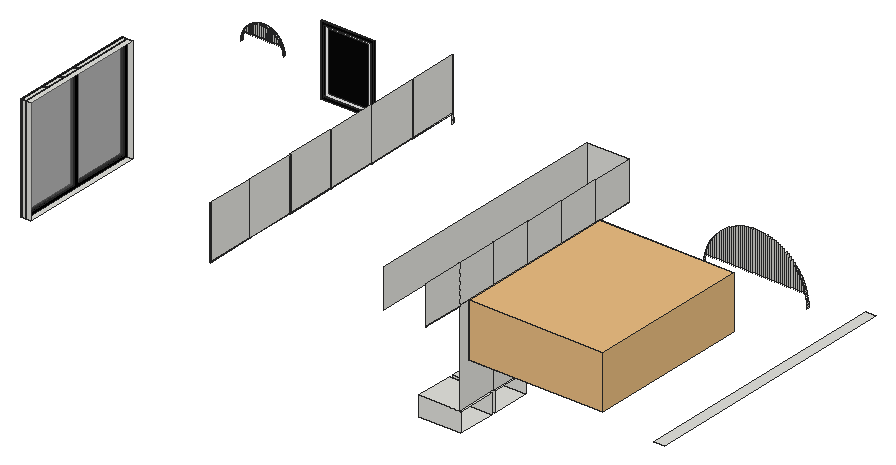
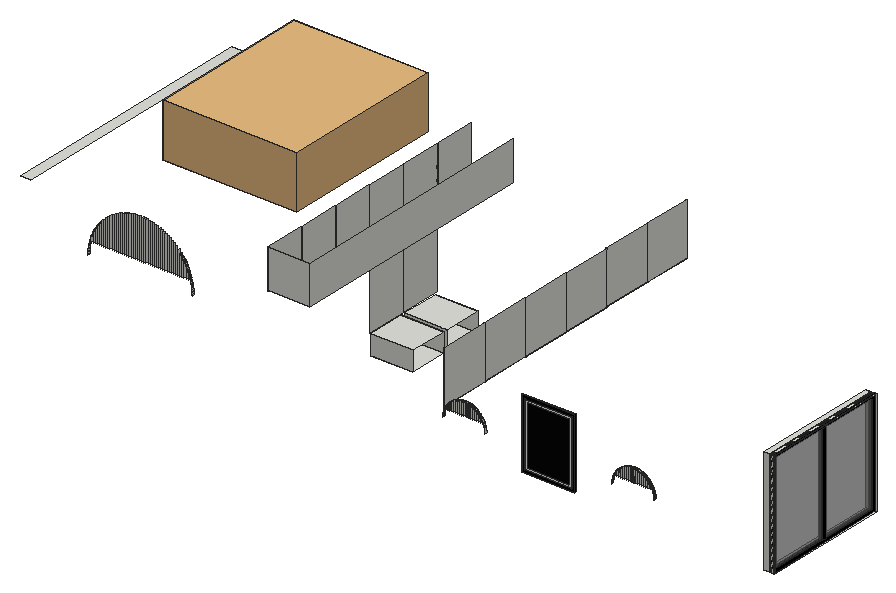
# SketchUp Ruby script. Lengths in inches.
U = 1.inch
M = Sketchup.active_model
def pt(a) = Geom::Point3d.new(a.map { |v| v * U })
def face(e, loops, mat)
  f = e.add_face(loops[0].map { |a| pt(a) })
  loops[1..].each { |l| e.add_face(l.map { |a| pt(a) }).erase! }
  f.material = f.back_material = mat if mat
  f
end
# faces: each face lists its corners as indices into pts; further lists are holes
def faces(e, pts, list, mat = nil) = list.each { |f| face(e, (f[0].is_a?(Array) ? f : [f]).map { |l| l.map { |i| pts[i] } }, mat) }
# xy, xz, yz: faces in a plane at the given z, y or x. An outline is a flat list of corners, or four numbers for a rectangle; further outlines are holes
def ring(l) = l.size == 4 ? [[l[0], l[1]], [l[2], l[1]], [l[2], l[3]], [l[0], l[3]]] : l.each_slice(2).to_a
def flat(e, list, mat, &to3) = list.each { |f| face(e, (f[0].is_a?(Array) ? f : [f]).map { |l| ring(l).map { |u, v| to3.(u, v) } }, mat) }
def xy(e, z, list, mat = nil) = flat(e, list, mat) { |x, y| [x, y, z] }
def xz(e, y, list, mat = nil) = flat(e, list, mat) { |x, z| [x, y, z] }
def yz(e, x, list, mat = nil) = flat(e, list, mat) { |y, z| [x, y, z] }
def lines(e, pts, list) = list.each { |a, b| e.add_line(pt(pts[a]), pt(pts[b])) }
# prism: a flat outline (further loops are holes) pulled along v
def prism(e, loops, v, mat = nil)
  f = face(e, loops, mat); d = Geom::Vector3d.new(v.map { |x| x * U })
  f.pushpull(f.normal.samedirection?(d) ? d.length : -d.length)
end
def box(e, o, s, mat = nil) = prism(e, [[o, [o[0] + s[0], o[1], o[2]], [o[0] + s[0], o[1] + s[1], o[2]], [o[0], o[1] + s[1], o[2]]]], [0, 0, s[2]], mat)
def at(x, y, z, deg = 0) = Geom::Transformation.translation(pt([x, y, z])) * Geom::Transformation.rotation(ORIGIN, Z_AXIS, deg.degrees)
def axes(o, x, y, z) = Geom::Transformation.new([*x, 0, *y, 0, *z, 0, *pt(o).to_a, 1])
def part(name) = M.definitions.add(name)
# library, detail: a bought-in or finely detailed component or shape, given as its bounding box
def library(name, o, s) = part(name).tap { |d| box(d.entities, o, s) }
def detail(e, o, s) = box(e.add_group.entities, o, s)
def put(e, d, t, mat = nil) = e.add_instance(d, t).tap { |i| i.material = mat if mat }
def group(e, t, mat = nil) = e.add_group.tap { |g| g.transformation = t; g.material = mat if mat }.entities
root = M.entities
M.materials.add("Plastic_Metalic_Black").color = [8, 8, 8]
M.materials.add("[Color M00]1").color = [254, 254, 254]
M.materials.add("[Color_008]").color = [30, 30, 30]
M.materials.add("[Color_009]").color = [0, 0, 0]
M.materials.add("[Translucent_Glass_Gray]").color = [128, 128, 128]
M.materials["[Translucent_Glass_Gray]"].alpha = 0.5
c1 = part("Photos Gallery Wall")
g1 = group(c1.entities,at(0,0,0))
xy(g1,23.66,[[13.71,0.34,13.7,1.03,31.9375,1.12,31.94,0.43]],"Plastic_Metalic_Black")
xy(g1,24.66,[[14.71,0.34,30.94,0.42,30.9375,1.02,14.7,0.94]],"Plastic_Metalic_Black")
xy(g1,48.82,[[14.71,0.34,14.7,0.94,30.9375,1.02,30.94,0.42]],"Plastic_Metalic_Black")
xy(g1,49.82,[[13.71,0.34,31.94,0.43,31.9375,1.12,13.7,1.03]],"Plastic_Metalic_Black")
p = [[13.7,1.03,49.82],[13.7,1.03,23.66],[13.71,0.34,23.66],[13.71,0.34,49.82],[31.94,0.43,23.66],[31.94,0.43,49.82],
  [30.94,0.42,24.66],[14.71,0.34,24.66],[14.71,0.34,48.82],[30.94,0.42,48.82],[31.9375,1.12,23.66],[31.9375,1.12,49.82],
  [14.7,1.04,24.66],[30.9375,1.11,24.66],[30.9375,1.11,48.82],[14.7,1.04,48.82],[14.7,0.94,48.82],[14.7,0.94,24.66],
  [30.9375,1.02,24.66],[30.9375,1.02,48.82],[29.9375,1.02,47.82],[29.9375,1.02,25.66],[15.7,0.95,25.66],[15.7,0.95,47.82]]
faces(g1,p,[[0,1,2,3],[[4,5,3,2],[6,7,8,9]],[10,11,5,4],[[11,10,1,0],[12,13,14,15]],[16,8,7,17],[18,6,9,19],[21,20,23,22]],"Plastic_Metalic_Black")
faces(g1,p,[[[17,18,19,16],[20,21,22,23]]],"[Color M00]1")
lines(g1,p,[[14,19],[15,16],[12,17],[13,18]])
c2 = part("Photo+Frames+03")
put(c2.entities,c1,axes([128.61,79.32,-32.19],[1.3608,0,0],[0,1.3608,0],[0,0,1.3608]))
c3 = library("ceiling fan",[0,0,0],[76.25,93.13,30.02])
xy(root,30.7,[[245.003,91.2,268.823,112.8],[245.003,115.2,268.823,136.8]])
xy(root,36,[[0,114.57,6,186.57]])
xy(root,41.7,[[245.003,91.2,268.823,112.8],[245.003,115.2,268.823,136.8]])
xy(root,88.8,[[150,61.77,150.18,89.203],[150,89.603,150.18,118.037],[150,118.437,150.18,146.87],[150,147.27,150.18,175.703],[150,176.103,150.18,204.537],
  [150,204.937,150.18,233.37]])
xy(root,89.2,[[150,61.77,150.18,89.203],[150,89.603,150.18,118.037],[150,118.437,150.18,146.87],[150,147.27,150.18,175.703],[150,176.103,150.18,204.537],
  [150,204.937,150.18,233.37]])
xy(root,95.8,[[268.823,66.2,269.003,89.8],[268.823,138.2,269.003,161.8],[268.823,162.2,269.003,185.8],[268.823,186.2,269.003,209.8]])
xy(root,96,[[413.003,48,419.003,198],[0,114.57,6,186.57]])
xy(root,96.2,[[268.823,66.2,269.003,89.8],[268.823,90.2,269.003,113.8],[268.823,114.2,269.003,137.8],[268.823,138.2,269.003,161.8],[268.823,162.2,269.003,185.8],
  [268.823,186.2,269.003,209.8]])
xz(root,61.77,[[150,89.2,150.18,118.8]])
xz(root,66.2,[[268.823,96.2,269.003,117.8]])
xz(root,89.203,[[150,89.2,150.18,118.8]])
xz(root,89.603,[[150,89.2,150.18,118.8]])
xz(root,89.8,[[268.823,96.2,269.003,117.8]])
xz(root,90.2,[[268.823,96.2,269.003,117.8]])
xz(root,91.2,[[245.003,30.7,268.823,41.7]])
xz(root,112.8,[[245.003,30.7,268.823,41.7]])
xz(root,113.8,[[268.823,96.2,269.003,117.8]])
xz(root,114.2,[[268.823,96.2,269.003,117.8]])
xz(root,114.57,[[0,36,6,96]])
xz(root,115.2,[[245.003,30.7,268.823,41.7]])
xz(root,118.037,[[150,89.2,150.18,118.8]])
xz(root,118.437,[[150,89.2,150.18,118.8]])
xz(root,136.8,[[245.003,30.7,268.823,41.7]])
xz(root,137.8,[[268.823,96.2,269.003,117.8]])
xz(root,138.2,[[268.823,96.2,269.003,117.8]])
xz(root,146.87,[[150,89.2,150.18,118.8]])
xz(root,147.27,[[150,89.2,150.18,118.8]])
xz(root,161.8,[[268.823,96.2,269.003,117.8]])
xz(root,162.2,[[268.823,96.2,269.003,117.8]])
xz(root,175.703,[[150,89.2,150.18,118.8]])
xz(root,176.103,[[150,89.2,150.18,118.8]])
xz(root,185.8,[[268.823,96.2,269.003,117.8]])
xz(root,186.2,[[268.823,96.2,269.003,117.8]])
xz(root,186.57,[[0,36,6,96]])
xz(root,204.537,[[150,89.2,150.18,118.8]])
xz(root,204.937,[[150,89.2,150.18,118.8]])
xz(root,209.8,[[268.823,96.2,269.003,117.8]])
xz(root,210,[[245.003,96,268.823,118]])
xz(root,233.37,[[150,84,150.18,88.8],[150,89.2,150.18,118.8]])
xz(root,233.57,[[150,84,150.18,119]])
xz(root,234.57,[[126,84,126.409,87.106,126.332,86.801,126.262,86.495,126.201,86.187,126.148,85.877,126.103,85.566,126.066,85.254,126.037,84.942,126.016,84.628,126.004,84.314],[126.409,87.106,127,88.533,127,88.794,126.913,88.592,126.797,88.3,126.688,88.006,126.587,87.708,126.494,87.408],[127,88.533,127.2,89.016,127.2,89.229,127.169,89.166,127.037,88.881,127,88.794],[127.2,89.016,127.608,90,128.2,90.772,128.2,90.924,128.11,90.797,127.936,90.536,127.768,90.27,127.608,90,127.454,89.726,127.308,89.448,127.2,89.229],[128.2,90.772,128.4,91.033,128.4,91.198,128.292,91.053,128.2,90.924],
  [128.4,91.033,129.4,92.336,129.4,92.368,129.296,92.26,129.082,92.03,128.875,91.793,128.674,91.552,128.48,91.305,128.4,91.198],[129.6,92.551,130.6,93.318,130.6,93.445,130.448,93.326,130.207,93.125,129.97,92.918,129.74,92.704,129.6,92.568],[130.6,93.318,130.8,93.472,130.8,93.599,130.695,93.52,130.6,93.445]])
yz(root,32.2,[[233.57,88.794,234.57,90.924]])
yz(root,32.4,[[233.57,89.229,234.57,91.198]])
yz(root,33.4,[[233.57,88.794,234.57,90.924],[233.57,90.924,234.57,92.368]])
yz(root,33.6,[[233.57,89.229,234.57,92.568]])
yz(root,34.6,[[233.57,88.794,234.57,89.229],[233.57,89.229,234.57,93.423],[233.57,93.423,234.57,93.445]])
yz(root,34.8,[[233.57,89.229,234.57,93.52],[233.57,93.52,234.57,93.599]])
yz(root,35.8,[[233.57,88.794,234.57,94.273]])
yz(root,36,[[233.57,89.229,234.57,94.392]])
yz(root,37,[[233.57,88.794,234.57,94.908]])
yz(root,37.2,[[233.57,89.229,234.57,94.997]])
yz(root,38.2,[[233.57,88.794,234.57,95.382]])
yz(root,38.4,[[233.57,89.229,234.57,95.446]])
yz(root,39.4,[[233.57,88.794,234.57,95.714]])
yz(root,39.6,[[233.57,89.229,234.57,95.757]])
yz(root,40.6,[[233.57,88.794,234.57,95.917]])
yz(root,41.8,[[233.57,88.794,234.57,95.997]])
yz(root,42,[[233.57,89.229,234.57,89.417],[233.57,89.417,234.57,96]])
yz(root,43,[[233.57,88.794,234.57,88.981],[233.57,88.981,234.57,95.958]])
yz(root,43.2,[[233.57,89.229,234.57,89.417],[233.57,89.417,234.57,95.939]])
yz(root,45.6,[[233.57,89.229,234.57,95.446]])
yz(root,48,[[233.57,89.229,234.57,94.392]])
yz(root,50.2,[[233.57,88.794,234.57,92.76]])
yz(root,50.4,[[233.695,89.229,234.57,92.568]])
yz(root,51.4,[[233.695,88.794,234.57,91.458]])
yz(root,51.6,[[233.695,89.229,234.57,91.198]])
yz(root,52.6,[[233.695,88.794,234.57,89.623]])
yz(root,128.2,[[233.57,88.794,234.57,90.772]])
yz(root,128.4,[[233.57,89.229,234.57,91.033]])
yz(root,129.4,[[233.57,88.794,234.57,90.924],[233.57,90.924,234.57,92.336]])
yz(root,129.6,[[233.57,89.229,234.57,92.551]])
yz(root,130.6,[[233.57,88.794,234.57,89.229],[233.57,89.229,234.57,93.318]])
yz(root,130.8,[[233.57,89.229,234.57,93.472],[233.57,93.472,234.57,93.52],[233.57,93.52,234.57,93.599]])
yz(root,131.8,[[233.57,88.794,234.57,94.273]])
yz(root,132,[[233.57,89.229,234.57,94.392]])
yz(root,133,[[233.57,88.794,234.57,94.908]])
yz(root,133.2,[[233.57,89.229,234.57,94.997]])
yz(root,134.2,[[233.57,88.794,234.57,95.382]])
yz(root,134.4,[[233.57,89.229,234.57,95.446]])
yz(root,135.4,[[233.57,88.794,234.57,95.714]])
yz(root,135.6,[[233.57,89.229,234.57,95.757]])
yz(root,136.6,[[233.57,88.794,234.57,95.917]])
yz(root,137.8,[[233.57,88.794,234.57,95.997]])
yz(root,138,[[233.57,89.229,234.57,89.417],[233.57,89.417,234.57,96]])
yz(root,139,[[233.57,88.794,234.57,88.981],[233.57,88.981,234.57,95.958]])
yz(root,139.2,[[233.57,89.229,234.57,89.417],[233.57,89.417,234.57,95.939]])
yz(root,141.6,[[233.57,89.229,234.57,95.446]])
yz(root,144,[[233.57,89.229,234.57,94.392]])
yz(root,146.2,[[233.57,88.794,234.57,92.76]])
yz(root,146.4,[[233.57,89.229,234.57,92.568]])
yz(root,147.4,[[233.57,88.794,234.57,91.458]])
yz(root,147.6,[[233.57,89.229,234.57,91.198]])
yz(root,148.6,[[233.57,88.794,234.57,89.623]])
yz(root,150,[[61.77,89.2,89.203,118.8],[89.603,89.2,118.037,118.8],[118.437,89.2,146.87,118.8],[147.27,89.2,175.703,118.8],[176.103,89.2,204.537,118.8],
  [204.937,89.2,233.37,118.8]])
yz(root,245.003,[[66,96,210,118]])
yz(root,268.823,[[90.2,42.7,113.8,95.8],[114.2,42.7,137.8,95.8]])
yz(root,269.003,[[66.2,96.2,89.8,117.8],[90.2,96.2,113.8,117.8],[114.2,96.2,137.8,117.8],[138.2,96.2,161.8,117.8],[162.2,96.2,185.8,117.8],
  [186.2,96.2,209.8,117.8]])
yz(root,313.953,[[209,85.483,210,89.103]])
yz(root,315.153,[[209,85.483,210,91.7]])
yz(root,316.353,[[208.6875,85.483,210,93.787]])
yz(root,317.553,[[209,85.483,210,95.548]])
yz(root,318.753,[[209,85.483,210,97.071]])
yz(root,319.953,[[209,85.483,210,98.413]])
yz(root,321.153,[[209,85.483,210,99.602]])
yz(root,322.353,[[209,85.483,210,100.667]])
yz(root,323.553,[[209,85.483,210,101.623]])
yz(root,324.753,[[209,85.483,210,102.484]])
yz(root,325.953,[[209,85.483,210,103.259]])
yz(root,327.153,[[209,85.483,210,103.954]])
yz(root,328.353,[[209,85.483,210,104.576]])
yz(root,329.553,[[209,85.483,210,105.132]])
yz(root,330.753,[[209,85.483,210,105.627]])
yz(root,331.953,[[209,85.483,210,106.058]])
yz(root,333.153,[[209,85.483,210,106.434]])
yz(root,334.353,[[209,85.483,210,106.755]])
yz(root,335.553,[[209,85.483,210,107.022]])
yz(root,336.753,[[209,85.483,210,107.24]])
yz(root,337.953,[[209,85.483,210,107.403]])
yz(root,339.153,[[209,85.483,210,107.521]])
yz(root,340.353,[[209,85.483,210,107.586]])
yz(root,341.553,[[209,85.483,210,107.605]])
yz(root,342.753,[[209,85.483,210,107.574]])
yz(root,343.953,[[209,85.483,210,107.494]])
yz(root,345.153,[[209,85.483,210,107.366]])
yz(root,346.353,[[209,85.483,210,107.186]])
yz(root,347.553,[[209,85.483,210,106.959]])
yz(root,348.753,[[209,85.483,210,106.676]])
yz(root,349.953,[[209,85.483,210,106.342]])
yz(root,351.153,[[209,85.483,210,105.951]])
yz(root,352.353,[[209,85.483,210,105.502]])
yz(root,353.553,[[209,85.483,210,104.994]])
yz(root,354.753,[[209,85.483,210,104.421]])
yz(root,355.953,[[209,85.483,210,103.778]])
yz(root,357.153,[[209,85.483,210,103.0625]])
yz(root,358.353,[[209,85.483,210,102.267]])
yz(root,359.553,[[209,85.483,210,101.383]])
yz(root,360.753,[[209,85.483,210,100.4]])
yz(root,361.953,[[209,85.483,210,99.304]])
yz(root,363.153,[[209,85.483,210,98.076]])
yz(root,364.353,[[209,85.483,210,96.695]])
yz(root,365.553,[[209,85.483,210,95.113]])
yz(root,366.753,[[209,85.483,210,93.28]])
yz(root,367.953,[[209,85.483,210,91.082]])
yz(root,369.153,[[209,85.483,210,88.294]])
p = [[371.003,210,78],[370.993,210,78.775],[370.993,208.875,78.775],[371.003,208.875,78],[311.8,210,78.775],[311.79,210,78],
  [311.79,209,78],[311.8,209,78.775],[370.962,210,79.549],[370.962,208.875,79.549],[311.83,210,79.549],[311.83,209,79.549],
  [370.912,210,80.323],[370.912,208.875,80.323],[311.881,210,80.323],[311.881,209,80.323],[370.841,210,81.095],[370.841,208.875,81.095],
  [311.952,210,81.095],[311.952,209,81.095],[370.75,210,81.864],[370.75,208.875,81.864],[312.043,210,81.864],[312.043,209,81.864],
  [370.639,210,82.631],[370.639,208.875,82.631],[312.154,210,82.631],[312.154,209,82.631],[370.553,210,83.129],[370.553,208.875,83.129],
  [312.286,210,83.395],[312.286,209,83.395],[312.437,210,84.156],[312.437,209,84.156],[30.004,234.57,84.314],[30,234.57,84],
  [30,233.57,84],[30.004,233.57,84.314],[126.409,234.57,87.106],[126,234.57,84],[126,233.57,84],[126.409,233.57,87.106],
  [150,234.57,84],[149.996,234.57,84.314],[149.996,233.57,84.314],[150,233.57,84],[54,234.57,84],[53.996,234.57,84.314],
  [53.996,233.695,84.314],[54,233.695,84],[370.353,210,84.169],[370.185,210,84.912],[370.185,208.875,84.912],[370.353,208.875,84.169],
  [312.608,210,84.912],[312.608,209,84.912],[30.016,234.57,84.628],[30.016,233.57,84.628],[149.984,234.57,84.628],[149.984,233.57,84.628],
  [53.984,234.57,84.628],[53.984,233.695,84.628],[30.037,234.57,84.942],[30.037,233.57,84.942],[149.963,234.57,84.942],[149.963,233.57,84.942],
  [53.963,234.57,84.942],[53.963,233.695,84.942],[369.994,210,85.663],[369.994,208.875,85.663],[312.753,210,85.483],[312.753,209,85.483],
  [30.066,234.57,85.254],[30.066,233.57,85.254],[149.934,234.57,85.254],[149.934,233.57,85.254],[53.934,234.57,85.254],[53.934,233.695,85.254],
  [30.103,234.57,85.566],[30.103,233.57,85.566],[149.897,234.57,85.566],[149.897,233.57,85.566],[53.897,234.57,85.566],[53.897,233.695,85.566],
  [30.148,234.57,85.877],[30.148,233.57,85.877],[149.852,234.57,85.877],[149.852,233.57,85.877],[53.852,234.57,85.877],[53.852,233.695,85.877],
  [369.784,210,86.409],[369.784,208.875,86.409],[30.201,234.57,86.187],[30.201,233.57,86.187],[149.799,234.57,86.187],[149.799,233.57,86.187],
  [53.799,234.57,86.187],[53.799,233.695,86.187],[313.009,210,86.409],[312.953,210,86.21],[312.953,209,86.21],[313.009,209,86.409],
  [30.262,234.57,86.495],[30.262,233.57,86.495],[149.738,234.57,86.495],[149.738,233.57,86.495],[53.738,234.57,86.495],[53.738,233.695,86.495],
  [369.554,210,87.149],[369.554,208.875,87.149],[313.239,210,87.149],[313.239,209,87.149],[30.332,234.57,86.801],[30.332,233.57,86.801],
  [149.668,234.57,86.801],[149.668,233.57,86.801],[53.668,234.57,86.801],[53.668,233.695,86.801],[30.409,234.57,87.106],[30.409,233.57,87.106],
  [149.591,234.57,87.106],[149.591,233.57,87.106],[53.591,234.57,87.106],[53.591,233.695,87.106],[369.353,210,87.741],[369.353,208.875,87.741],
  [313.488,210,87.883],[313.488,209,87.883],[30.494,234.57,87.408],[30.494,233.57,87.408],[127,234.57,88.533],[127,233.57,88.533],
  [149.506,234.57,87.408],[149.506,233.57,87.408],[53.506,234.57,87.408],[53.506,233.695,87.408],[30.587,234.57,87.708],[30.587,233.57,87.708],
  [149.413,234.57,87.708],[149.413,233.57,87.708],[53.413,234.57,87.708],[53.413,233.695,87.708],[30.688,234.57,88.006],[30.688,233.57,88.006],
  [149.312,234.57,88.006],[149.312,233.57,88.006],[53.312,234.57,88.006],[53.312,233.695,88.006],[313.756,210,88.61],[313.756,209,88.61],
  [30.797,234.57,88.3],[30.797,233.57,88.3],[149.203,234.57,88.3],[149.203,233.57,88.3],[53.203,234.57,88.3],[53.203,233.695,88.3],
  [369.153,210,88.294],[369.037,210,88.61],[369.037,209,88.61],[369.153,209,88.294],[30.913,234.57,88.592],[30.913,233.57,88.592],
  [149.087,234.57,88.592],[149.087,233.57,88.592],[53.087,234.57,88.592],[53.087,233.695,88.592],[313.953,210,89.103],[313.953,209,89.103],
  [368.749,210,89.33],[368.749,209,89.33],[31,234.57,88.794],[31,233.57,88.794],[148.963,234.57,88.881],[148.963,233.57,88.881],
  [52.963,234.57,88.881],[52.963,233.695,88.881],[44.2,234.57,88.794],[44.187,234.57,95.799],[44.187,233.57,95.799],[44.2,233.57,88.794],
  [45.4,234.57,88.794],[45.408,234.57,95.506],[45.408,233.57,95.506],[45.4,233.57,88.794],[46.6,234.57,88.794],[46.592,234.57,95.087],
  [46.592,233.57,95.087],[46.6,233.57,88.794],[47.8,234.57,88.794],[47.726,234.57,94.546],[47.726,233.57,94.546],[47.8,233.57,88.794],
  [49,234.57,88.794],[49.053,234.57,93.708],[49.053,233.57,93.708],[49,233.57,88.794],[140.2,234.57,88.794],[140.187,234.57,95.799],
  [140.187,233.57,95.799],[140.2,233.57,88.794],[141.4,234.57,88.794],[141.408,234.57,95.506],[141.408,233.57,95.506],[141.4,233.57,88.794],
  [142.6,234.57,88.794],[142.592,234.57,95.087],[142.592,233.57,95.087],[142.6,233.57,88.794],[143.8,234.57,88.794],[143.726,234.57,94.546],
  [143.726,233.57,94.546],[143.8,233.57,88.794],[145,234.57,88.794],[145.053,234.57,93.708],[145.053,233.57,93.708],[145,233.57,88.794],
  [148.831,234.57,89.166],[148.831,233.57,89.166],[52.831,234.57,89.166],[52.831,233.695,89.166],[127.608,234.57,90],[127.2,234.57,89.016],
  [127.2,233.57,89.016],[127.608,233.57,90],[31.308,234.57,89.448],[31.2,234.57,89.229],[31.2,233.57,89.229],[31.308,233.57,89.448],
  [40.746,234.57,95.934],[40.8,234.57,89.229],[40.8,233.57,89.229],[40.746,233.57,95.934],[44.388,234.57,95.759],[44.4,234.57,89.229],
  [44.4,233.57,89.229],[44.388,233.57,95.759],[46.793,234.57,95],[46.8,234.57,89.229],[46.8,233.57,89.229],[46.793,233.57,95],
  [49.305,234.57,93.52],[49.2,234.57,89.229],[49.2,233.57,89.229],[49.305,233.57,93.52],[136.746,234.57,95.934],[136.8,234.57,89.229],
  [136.8,233.57,89.229],[136.746,233.57,95.934],[140.388,234.57,95.759],[140.4,234.57,89.229],[140.4,233.57,89.229],[140.388,233.57,95.759],
  [142.793,234.57,95],[142.8,234.57,89.229],[142.8,233.57,89.229],[142.793,233.57,95],[145.305,234.57,93.52],[145.2,234.57,89.229],
  [145.2,233.57,89.229],[145.305,233.57,93.52],[148.8,234.57,89.229],[148.8,233.57,89.229],[52.8,234.57,89.229],[52.8,233.695,89.229],
  [368.443,210,90.042],[368.443,209,90.042],[31.454,234.57,89.726],[31.454,233.57,89.726],[314.349,210,90.042],[314.153,210,89.585],
  [314.153,209,89.585],[314.349,209,90.042],[148.6,234.57,89.623],[148.546,234.57,89.726],[148.546,233.57,89.726],[148.6,233.57,89.623],
  [52.6,234.57,89.623],[52.546,234.57,89.726],[52.546,233.695,89.726],[52.6,233.695,89.623],[31.608,234.57,90],[31.608,233.57,90],
  [148.392,234.57,90],[148.392,233.57,90],[52.392,234.57,90],[52.392,233.695,90],[314.674,210,90.746],[314.674,209,90.746],
  [368.153,210,90.672],[368.153,209,90.672],[31.768,234.57,90.27],[31.768,233.57,90.27],[128.2,234.57,90.772],[128.2,233.57,90.772],
  [148.232,234.57,90.27],[148.232,233.57,90.27],[52.232,234.57,90.27],[52.232,233.695,90.27],[31.936,234.57,90.536],[31.936,233.57,90.536],
  [148.064,234.57,90.536],[148.064,233.57,90.536],[52.064,234.57,90.536],[52.064,233.695,90.536],[32.11,234.57,90.797],[32.11,233.57,90.797],
  [147.89,234.57,90.797],[147.89,233.57,90.797],[51.89,234.57,90.797],[51.89,233.695,90.797],[315.017,210,91.441],[315.017,209,91.441],
  [32.2,234.57,90.924],[32.2,233.57,90.924],[147.708,234.57,91.053],[147.708,233.57,91.053],[51.708,234.57,91.053],[51.708,233.695,91.053],
  [129.4,234.57,92.336],[128.4,234.57,91.033],[128.4,233.57,91.033],[129.4,233.57,92.336],[367.953,210,91.082],[367.776,210,91.441],
  [367.776,209,91.441],[367.953,209,91.082],[147.6,234.57,91.198],[147.6,233.57,91.198],[51.6,234.57,91.198],[51.6,233.695,91.198],
  [32.48,234.57,91.305],[32.4,234.57,91.198],[32.4,233.57,91.198],[32.48,233.57,91.305],[32.674,234.57,91.552],[32.674,233.57,91.552],
  [315.153,210,91.7],[315.153,209,91.7],[367.415,210,92.127],[367.415,209,92.127],[147.4,234.57,91.458],[147.326,234.57,91.552],
  [147.326,233.57,91.552],[147.4,233.57,91.458],[51.4,234.57,91.458],[51.326,234.57,91.552],[51.326,233.695,91.552],[51.4,233.695,91.458],
  [32.875,234.57,91.793],[32.875,233.57,91.793],[147.125,234.57,91.793],[147.125,233.57,91.793],[51.125,234.57,91.793],[51.125,233.695,91.793],
  [33.082,234.57,92.03],[33.082,233.57,92.03],[146.918,234.57,92.03],[146.918,233.57,92.03],[50.918,234.57,92.03],[50.918,233.695,92.03],
  [33.296,234.57,92.26],[33.296,233.57,92.26],[146.704,234.57,92.26],[146.704,233.57,92.26],[50.704,234.57,92.26],[50.704,233.695,92.26],
  [315.378,210,92.127],[315.353,210,92.08],[315.353,208.6875,92.08],[315.378,208.6875,92.127],[315.756,210,92.803],[315.756,208.6875,92.803],
  [367.037,210,92.803],[367.037,209,92.803],[33.4,234.57,92.368],[33.4,233.57,92.368],[146.485,234.57,92.485],[146.485,233.57,92.485],
  [50.485,234.57,92.485],[50.485,233.695,92.485],[146.4,234.57,92.568],[146.4,233.57,92.568],[50.4,234.57,92.568],[50.4,233.695,92.568],
  [33.74,234.57,92.704],[33.6,234.57,92.568],[33.6,233.57,92.568],[33.74,233.57,92.704],[130.6,234.57,93.318],[129.6,234.57,92.551],
  [129.6,233.57,92.551],[130.6,233.57,93.318],[33.97,234.57,92.918],[33.97,233.57,92.918],[316.153,210,93.469],[316.153,208.6875,93.469],
  [366.953,210,92.944],[366.953,209,92.944],[50.2,234.57,92.76],[50.03,234.57,92.918],[50.03,233.57,92.918],[50.2,233.57,92.76],
  [146.2,234.57,92.76],[146.03,234.57,92.918],[146.03,233.57,92.918],[146.2,233.57,92.76],[34.207,234.57,93.125],[34.207,233.57,93.125],
  [49.793,234.57,93.125],[49.793,233.57,93.125],[145.793,234.57,93.125],[145.793,233.57,93.125],[34.448,234.57,93.326],[34.448,233.57,93.326],
  [49.552,234.57,93.326],[49.552,233.57,93.326],[145.552,234.57,93.326],[145.552,233.57,93.326],[366.753,210,93.28],[366.64,210,93.469],
  [366.64,209,93.469],[366.753,209,93.28],[34.6,234.57,93.445],[34.6,233.57,93.445],[316.353,210,93.787],[316.353,208.6875,93.787],
  [366.227,210,94.125],[366.227,209,94.125],[34.947,234.57,93.708],[34.8,234.57,93.599],[34.8,233.57,93.599],[34.947,233.57,93.708],
  [130.947,234.57,93.708],[130.8,234.57,93.599],[130.8,233.57,93.599],[130.947,233.57,93.708],[35.203,234.57,93.89],[35.203,233.57,93.89],
  [48.797,234.57,93.89],[48.797,233.57,93.89],[131.203,234.57,93.89],[131.203,233.57,93.89],[144.797,234.57,93.89],[144.797,233.57,93.89],
  [35.464,234.57,94.064],[35.464,233.57,94.064],[48.536,234.57,94.064],[48.536,233.57,94.064],[131.464,234.57,94.064],[131.464,233.57,94.064],
  [144.536,234.57,94.064],[144.536,233.57,94.064],[316.566,210,94.125],[316.553,210,94.104],[316.553,209,94.104],[316.566,209,94.125],
  [316.997,210,94.769],[316.997,209,94.769],[365.796,210,94.769],[365.796,209,94.769],[35.73,234.57,94.232],[35.73,233.57,94.232],
  [48.27,234.57,94.232],[48.27,233.57,94.232],[131.73,234.57,94.232],[131.73,233.57,94.232],[144.27,234.57,94.232],[144.27,233.57,94.232],
  [35.8,234.57,94.273],[35.8,233.57,94.273],[48,234.57,94.392],[48,233.57,94.392],[131.8,234.57,94.273],[131.8,233.57,94.273],
  [144,234.57,94.392],[144,233.57,94.392],[36.274,234.57,94.546],[36,234.57,94.392],[36,233.57,94.392],[36.274,233.57,94.546],
  [132.274,234.57,94.546],[132,234.57,94.392],[132,233.57,94.392],[132.274,233.57,94.546],[36.552,234.57,94.692],[36.552,233.57,94.692],
  [47.448,234.57,94.692],[47.448,233.57,94.692],[132.552,234.57,94.692],[132.552,233.57,94.692],[143.448,234.57,94.692],[143.448,233.57,94.692],
  [36.834,234.57,94.831],[36.834,233.57,94.831],[47.166,234.57,94.831],[47.166,233.57,94.831],[132.834,234.57,94.831],[132.834,233.57,94.831],
  [143.166,234.57,94.831],[143.166,233.57,94.831],[317.444,210,95.402],[317.444,209,95.402],[365.753,210,94.83],[365.753,209,94.83],
  [37,234.57,94.908],[37,233.57,94.908],[46.881,234.57,94.963],[46.881,233.57,94.963],[133,234.57,94.908],[133,233.57,94.908],
  [142.881,234.57,94.963],[142.881,233.57,94.963],[37.408,234.57,95.087],[37.2,234.57,94.997],[37.2,233.57,94.997],[37.408,233.57,95.087],
  [133.408,234.57,95.087],[133.2,234.57,94.997],[133.2,233.57,94.997],[133.408,233.57,95.087],[365.553,210,95.113],[365.349,210,95.402],
  [365.349,209,95.402],[365.553,209,95.113],[37.7,234.57,95.203],[37.7,233.57,95.203],[46.3,234.57,95.203],[46.3,233.57,95.203],
  [133.7,234.57,95.203],[133.7,233.57,95.203],[142.3,234.57,95.203],[142.3,233.57,95.203],[37.994,234.57,95.312],[37.994,233.57,95.312],
  [46.006,234.57,95.312],[46.006,233.57,95.312],[133.994,234.57,95.312],[133.994,233.57,95.312],[142.006,234.57,95.312],[142.006,233.57,95.312],
  [38.2,234.57,95.382],[38.2,233.57,95.382],[45.708,234.57,95.413],[45.708,233.57,95.413],[134.2,234.57,95.382],[134.2,233.57,95.382],
  [141.708,234.57,95.413],[141.708,233.57,95.413],[317.553,210,95.548],[317.553,209,95.548],[364.885,210,96.023],[364.885,209,96.023],
  [38.592,234.57,95.506],[38.4,234.57,95.446],[38.4,233.57,95.446],[38.592,233.57,95.506],[45.6,234.57,95.446],[45.6,233.57,95.446],
  [134.592,234.57,95.506],[134.4,234.57,95.446],[134.4,233.57,95.446],[134.592,233.57,95.506],[141.6,234.57,95.446],[141.6,233.57,95.446],
  [38.894,234.57,95.591],[38.894,233.57,95.591],[45.106,234.57,95.591],[45.106,233.57,95.591],[134.894,234.57,95.591],[134.894,233.57,95.591],
  [141.106,234.57,95.591],[141.106,233.57,95.591],[39.199,234.57,95.668],[39.199,233.57,95.668],[44.801,234.57,95.668],[44.801,233.57,95.668],
  [135.199,234.57,95.668],[135.199,233.57,95.668],[140.801,234.57,95.668],[140.801,233.57,95.668],[39.4,234.57,95.714],[39.4,233.57,95.714],
  [44.495,234.57,95.738],[44.495,233.57,95.738],[135.4,234.57,95.714],[135.4,233.57,95.714],[140.495,234.57,95.738],[140.495,233.57,95.738],
  [317.908,210,96.023],[317.753,210,95.816],[317.753,209,95.816],[317.908,209,96.023],[39.813,234.57,95.799],[39.6,234.57,95.757],
  [39.6,233.57,95.757],[39.813,233.57,95.799],[40.123,234.57,95.852],[40.123,233.57,95.852],[43.877,234.57,95.852],[43.877,233.57,95.852],
  [135.813,234.57,95.799],[135.6,234.57,95.757],[135.6,233.57,95.757],[135.813,233.57,95.799],[136.123,234.57,95.852],[136.123,233.57,95.852],
  [139.877,234.57,95.852],[139.877,233.57,95.852],[40.434,234.57,95.897],[40.434,233.57,95.897],[40.6,234.57,95.917],[40.6,233.57,95.917],
  [41.058,234.57,95.963],[41.058,233.57,95.963],[43.254,234.57,95.934],[43.2,234.57,95.939],[43.2,233.57,95.939],[43.254,233.57,95.934],
  [43.566,234.57,95.897],[43.566,233.57,95.897],[136.434,234.57,95.897],[136.434,233.57,95.897],[136.6,234.57,95.917],[136.6,233.57,95.917],
  [137.058,234.57,95.963],[137.058,233.57,95.963],[139.254,234.57,95.934],[139.2,234.57,95.939],[139.2,233.57,95.939],[139.254,233.57,95.934],
  [139.566,234.57,95.897],[139.566,233.57,95.897],[318.388,210,96.632],[318.388,209,96.632],[364.553,210,96.444],[364.553,209,96.444],
  [41.372,234.57,95.984],[41.372,233.57,95.984],[41.686,234.57,95.996],[41.686,233.57,95.996],[41.8,234.57,95.997],[41.8,233.57,95.997],
  [42.314,234.57,95.996],[42,234.57,96],[42,233.57,96],[42.314,233.57,95.996],[42.6,234.57,95.985],[42.6,233.57,95.985],
  [42.942,234.57,95.963],[42.628,234.57,95.984],[42.628,233.57,95.984],[42.942,233.57,95.963],[43,234.57,95.958],[43,233.57,95.958],
  [137.372,234.57,95.984],[137.372,233.57,95.984],[137.686,234.57,95.996],[137.686,233.57,95.996],[137.8,234.57,95.997],[137.8,233.57,95.997],
  [138.314,234.57,95.996],[138,234.57,96],[138,233.57,96],[138.314,233.57,95.996],[138.6,234.57,95.985],[138.6,233.57,95.985],
  [138.942,234.57,95.963],[138.628,234.57,95.984],[138.628,233.57,95.984],[138.942,233.57,95.963],[139,234.57,95.958],[139,233.57,95.958],
  [318.753,210,97.071],[318.753,209,97.071],[364.353,210,96.695],[363.909,210,97.228],[363.909,209,97.228],[364.353,209,96.695],
  [137.8,234.57,96],[129.4,234.57,92.368],[129.4,234.57,92.373],[43,234.57,95.997],[41.8,234.57,96],[33.4,234.57,92.373]]
faces(root,p,[[0,1,2,3],[4,5,6,7],[1,8,9,2],[10,4,7,11],[8,12,13,9],[14,10,11,15],[12,16,17,13],[18,14,15,19],
  [16,20,21,17],[22,18,19,23],[20,24,25,21],[26,22,23,27],[24,28,29,25],[30,26,27,31],[32,30,31,33],[34,35,36,37],
  [38,39,40,41],[42,43,44,45],[46,47,48,49],[50,51,52,53],[54,32,33,55],[56,34,37,57],[43,58,59,44],[47,60,61,48],
  [62,56,57,63],[58,64,65,59],[60,66,67,61],[51,68,69,52],[70,54,55,71],[72,62,63,73],[64,74,75,65],[66,76,77,67],
  [78,72,73,79],[74,80,81,75],[76,82,83,77],[84,78,79,85],[80,86,87,81],[82,88,89,83],[68,90,91,69],[92,84,85,93],
  [86,94,95,87],[88,96,97,89],[98,99,100,101],[102,92,93,103],[94,104,105,95],[96,106,107,97],[90,108,109,91],[110,98,101,111],
  [112,102,103,113],[104,114,115,105],[106,116,117,107],[118,112,113,119],[114,120,121,115],[116,122,123,117],[108,124,125,109],[126,110,111,127],
  [128,118,119,129],[130,38,41,131],[120,132,133,121],[122,134,135,123],[136,128,129,137],[132,138,139,133],[134,140,141,135],[142,136,137,143],
  [138,144,145,139],[140,146,147,141],[148,126,127,149],[150,142,143,151],[144,152,153,145],[146,154,155,147],[156,157,158,159],[160,150,151,161],
  [152,162,163,153],[154,164,165,155],[166,148,149,167],[157,168,169,158],[170,160,161,171],[162,172,173,163],[164,174,175,165],[176,177,178,179],
  [180,181,182,183],[184,185,186,187],[188,189,190,191],[192,193,194,195],[196,197,198,199],[200,201,202,203],[204,205,206,207],[208,209,210,211],
  [212,213,214,215],[172,216,217,173],[174,218,219,175],[220,221,222,223],[224,225,226,227],[228,229,230,231],[232,233,234,235],[236,237,238,239],
  [240,241,242,243],[244,245,246,247],[248,249,250,251],[252,253,254,255],[256,257,258,259],[216,260,261,217],[218,262,263,219],[168,264,265,169],
  [266,224,227,267],[268,269,270,271],[272,273,274,275],[276,277,278,279],[280,266,267,281],[273,282,283,274],[277,284,285,278],[286,268,271,287],
  [264,288,289,265],[290,280,281,291],[292,220,223,293],[282,294,295,283],[284,296,297,285],[298,290,291,299],[294,300,301,295],[296,302,303,297],
  [304,298,299,305],[300,306,307,301],[302,308,309,303],[310,286,287,311],[312,304,305,313],[306,314,315,307],[308,316,317,309],[318,319,320,321],
  [322,323,324,325],[314,326,327,315],[316,328,329,317],[330,331,332,333],[334,330,333,335],[336,310,311,337],[323,338,339,324],[340,341,342,343],
  [344,345,346,347],[348,334,335,349],[341,350,351,342],[345,352,353,346],[354,348,349,355],[350,356,357,351],[352,358,359,353],[360,354,355,361],
  [356,362,363,357],[358,364,365,359],[366,367,368,369],[370,366,369,371],[338,372,373,339],[374,360,361,375],[362,376,377,363],[364,378,379,365],
  [376,380,381,377],[378,382,383,379],[384,385,386,387],[388,389,390,391],[392,384,387,393],[394,370,371,395],[372,396,397,373],[398,399,400,401],
  [402,403,404,405],[406,392,393,407],[399,408,409,400],[403,410,411,404],[412,406,407,413],[408,414,415,409],[410,416,417,411],[418,419,420,421],
  [422,412,413,423],[414,240,243,415],[416,256,259,417],[424,394,395,425],[419,426,427,420],[428,429,430,431],[432,433,434,435],[436,428,431,437],
  [193,438,439,194],[440,432,435,441],[213,442,443,214],[444,436,437,445],[438,446,447,439],[448,440,441,449],[442,450,451,443],[452,453,454,455],
  [456,452,455,457],[426,458,459,427],[460,444,445,461],[446,462,463,447],[464,448,449,465],[450,466,467,451],[468,460,461,469],[462,470,471,463],
  [472,464,465,473],[466,474,475,467],[476,477,478,479],[480,481,482,483],[484,476,479,485],[189,486,487,190],[488,480,483,489],[209,490,491,210],
  [492,484,485,493],[486,494,495,487],[496,488,489,497],[490,498,499,491],[500,456,457,501],[458,502,503,459],[504,492,493,505],[494,506,507,495],
  [508,496,497,509],[498,510,511,499],[512,513,514,515],[506,236,239,507],[516,517,518,519],[510,252,255,511],[520,521,522,523],[524,512,515,525],
  [185,526,527,186],[528,516,519,529],[205,530,531,206],[532,524,525,533],[526,534,535,527],[536,528,529,537],[530,538,539,531],[540,532,533,541],
  [534,542,543,535],[544,536,537,545],[538,546,547,539],[548,500,501,549],[521,550,551,522],[552,553,554,555],[542,556,557,543],[558,559,560,561],
  [546,562,563,547],[564,552,555,565],[181,566,567,182],[568,558,561,569],[201,570,571,202],[572,564,565,573],[566,574,575,567],[576,568,569,577],
  [570,578,579,571],[580,572,573,581],[582,232,235,583],[574,582,583,575],[584,576,577,585],[586,248,251,587],[578,586,587,579],[588,589,590,591],
  [592,593,594,595],[596,592,595,597],[177,598,599,178],[600,601,602,603],[604,600,603,605],[197,606,607,198],[608,596,597,609],[610,608,609,611],
  [612,228,231,613],[614,615,616,617],[618,614,617,619],[598,618,619,599],[620,604,605,621],[622,620,621,623],[624,244,247,625],[626,627,628,629],
  [630,626,629,631],[606,630,631,607],[632,588,591,633],[550,634,635,551],[636,612,613,637],[638,636,637,639],[640,638,639,641],[642,643,644,645],
  [646,642,645,647],[648,649,650,651],[649,646,647,650],[652,648,651,653],[654,624,625,655],[656,654,655,657],[658,656,657,659],[660,661,662,663],
  [664,660,663,665],[666,667,668,669],[667,664,665,668],[670,666,669,671],[672,632,633,673],[674,675,676,677]])
lines(root,p,[[658,678],[679,680],[652,681],[640,682],[374,683]])
g2 = group(root,at(3,114.57,36))
xy(g2,0,[[-2.36,0,0,72]],"[Color_009]")
xy(g2,1.43,[[-2.36,1.71,-1.97,35.14],[-2.36,36.86,-1.97,70.29]])
xy(g2,1.43,[[-0.59,1.71,0,35.14],[-0.59,36.86,0,70.29]],"[Color_009]")
xy(g2,58.57,[[-2.36,1.71,-1.97,35.14],[-1.97,1.71,-0.59,35.14],[-0.59,1.71,0,35.14],[-2.36,36.86,-1.97,70.29],[-1.97,36.86,-0.59,70.29],
  [-0.59,36.86,0,70.29]])
xy(g2,60,[[-2.36,0,0,72]],"[Color_008]")
xz(g2,0,[[-2.36,0,0,60]],"[Color_009]")
xz(g2,1.71,[[-2.36,1.43,-1.97,58.57]])
xz(g2,1.71,[[-0.59,1.43,0,58.57]],"[Color_009]")
xz(g2,35.14,[[-2.36,1.43,-1.97,58.57],[-0.59,1.43,0,58.57]],"[Color_009]")
xz(g2,36.86,[[-2.36,1.43,-1.97,58.57],[-0.59,1.43,0,58.57]])
xz(g2,70.29,[[-2.36,1.43,-1.97,58.57],[-0.59,1.43,0,58.57]],"[Color_009]")
xz(g2,72,[[-2.36,0,0,60]],"[Color_009]")
yz(g2,-2.36,[[[0,0,72,60],[1.71,1.43,70.29,58.57]],[35.14,1.43,36.86,58.57]],"[Color_009]")
yz(g2,-1.97,[[1.71,1.43,35.14,58.57],[36.86,1.43,70.29,58.57]],"[Translucent_Glass_Gray]")
yz(g2,-0.59,[[1.71,1.43,35.14,58.57],[36.86,1.43,70.29,58.57]],"[Translucent_Glass_Gray]")
yz(g2,0,[[[0,0,72,60],[1.71,1.43,35.14,58.57],[36.86,1.43,70.29,58.57]]],"[Color_009]")
put(root,c2,axes([-102.13,152.73,71.11],[1.2096,0,0],[0,1,0],[0,0,1.11]))
put(root,c3,at(302.6,54.16,96.36))
